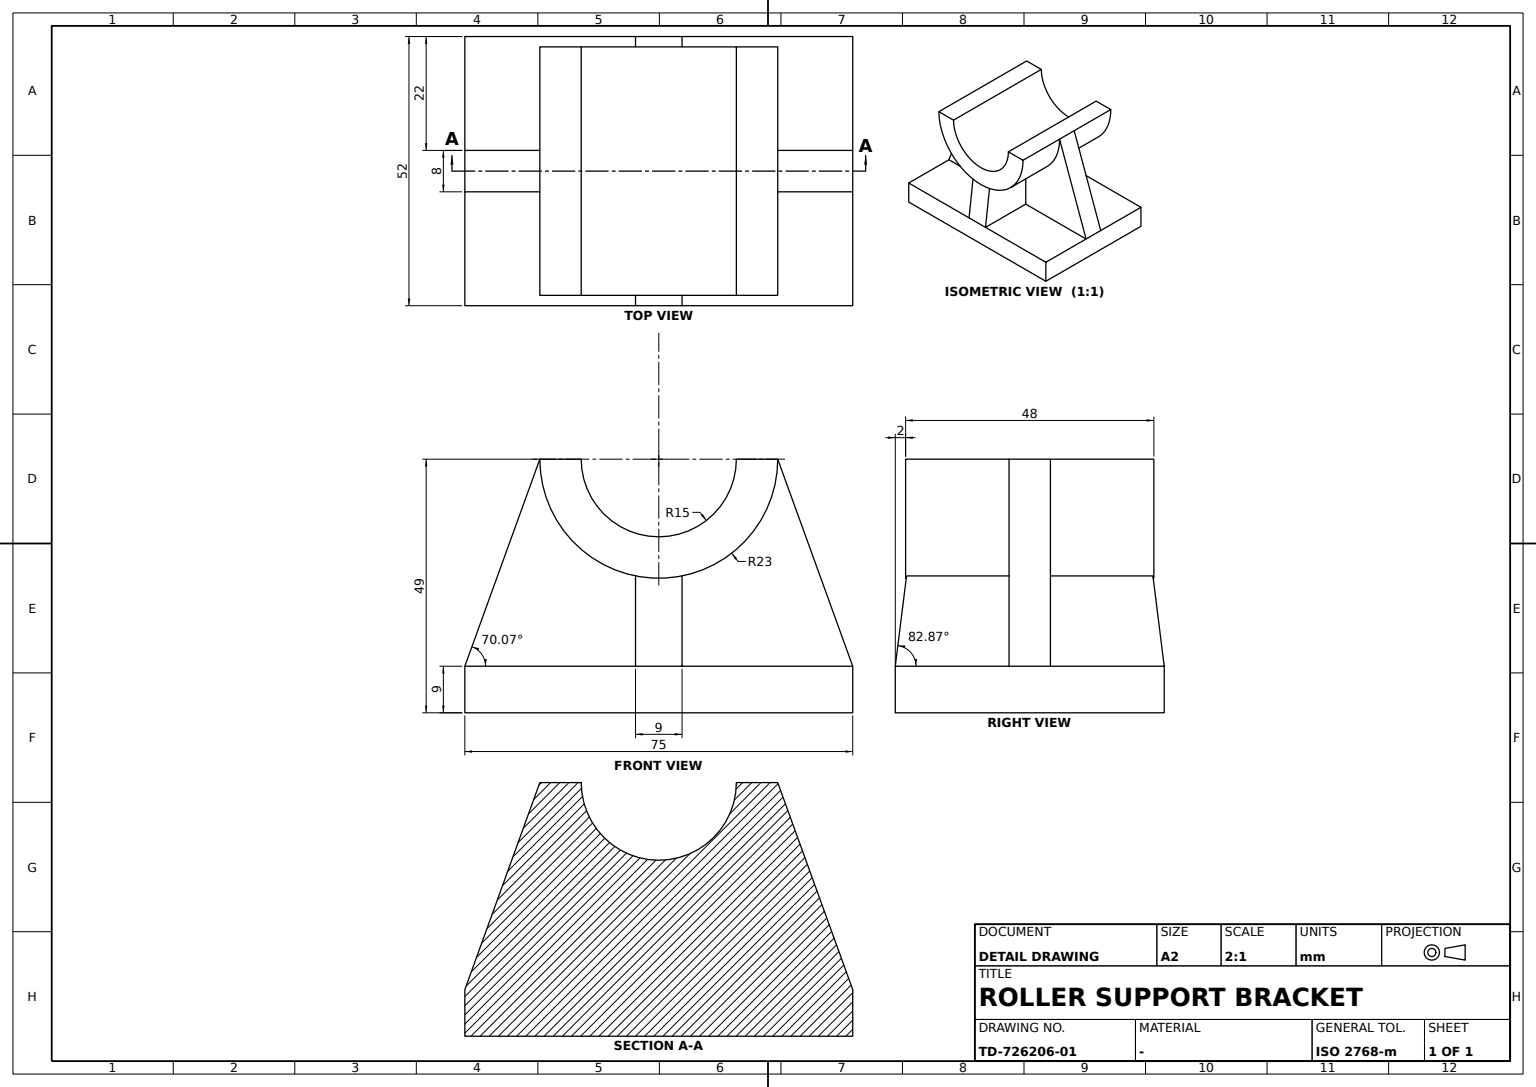
ISO-10303-21;
HEADER;
FILE_DESCRIPTION((''),'2;1');
FILE_NAME('','',(''),(''),'','','');
FILE_SCHEMA(('AUTOMOTIVE_DESIGN'));
ENDSEC;
DATA;
#1=APPLICATION_CONTEXT('');
#2=PRODUCT_CONTEXT('',#1,'mechanical');
#3=PRODUCT('','','',(#2));
#4=PRODUCT_DEFINITION_FORMATION('','',#3);
#5=PRODUCT_DEFINITION_CONTEXT('',#1,'design');
#6=PRODUCT_DEFINITION('','',#4,#5);
#7=PRODUCT_DEFINITION_SHAPE('','',#6);
#8=(LENGTH_UNIT()NAMED_UNIT(*)SI_UNIT(.MILLI.,.METRE.));
#9=(NAMED_UNIT(*)PLANE_ANGLE_UNIT()SI_UNIT($,.RADIAN.));
#10=(NAMED_UNIT(*)SI_UNIT($,.STERADIAN.)SOLID_ANGLE_UNIT());
#11=UNCERTAINTY_MEASURE_WITH_UNIT(LENGTH_MEASURE(0.005),#8,'distance_accuracy_value','');
#12=(GEOMETRIC_REPRESENTATION_CONTEXT(3)GLOBAL_UNCERTAINTY_ASSIGNED_CONTEXT((#11))GLOBAL_UNIT_ASSIGNED_CONTEXT((#8,#9,#10))REPRESENTATION_CONTEXT('',''));
#13=CARTESIAN_POINT('',(-4.,-37.5,4.5));
#14=VERTEX_POINT('',#13);
#15=CARTESIAN_POINT('',(4.,-37.5,4.5));
#16=VERTEX_POINT('',#15);
#17=CARTESIAN_POINT('',(0.,-37.5,4.5));
#18=DIRECTION('',(1.,0.,0.));
#19=VECTOR('',#18,1000.);
#20=LINE('',#17,#19);
#21=EDGE_CURVE('',#14,#16,#20,.T.);
#22=ORIENTED_EDGE('',*,*,#21,.T.);
#23=CARTESIAN_POINT('',(4.,-23.,44.5));
#24=VERTEX_POINT('',#23);
#25=CARTESIAN_POINT('',(4.,-34.586383,12.537564));
#26=DIRECTION('',(0.,-0.340799324,-0.940136065));
#27=VECTOR('',#26,1000.);
#28=LINE('',#25,#27);
#29=EDGE_CURVE('',#24,#16,#28,.T.);
#30=ORIENTED_EDGE('',*,*,#29,.F.);
#31=CARTESIAN_POINT('',(-4.,-23.,44.5));
#32=VERTEX_POINT('',#31);
#33=CARTESIAN_POINT('',(0.,-23.,44.5));
#34=LINE('',#33,#19);
#35=EDGE_CURVE('',#32,#24,#34,.T.);
#36=ORIENTED_EDGE('',*,*,#35,.F.);
#37=CARTESIAN_POINT('',(-4.,-34.586383,12.537564));
#38=LINE('',#37,#27);
#39=EDGE_CURVE('',#32,#14,#38,.T.);
#40=ORIENTED_EDGE('',*,*,#39,.T.);
#41=EDGE_LOOP('',(#22,#30,#36,#40));
#42=FACE_BOUND('',#41,.T.);
#43=DIRECTION('',(0.,-0.940136065,0.340799324));
#44=AXIS2_PLACEMENT_3D('',#33,#43,#26);
#45=PLANE('',#44);
#46=ADVANCED_FACE('',(#42),#45,.T.);
#47=CARTESIAN_POINT('',(24.,-15.,44.5));
#48=VERTEX_POINT('',#47);
#49=CARTESIAN_POINT('',(24.,15.,44.5));
#50=VERTEX_POINT('',#49);
#51=CARTESIAN_POINT('',(24.,0.,44.5));
#52=DIRECTION('',(0.,0.,-1.));
#53=AXIS2_PLACEMENT_3D('',#51,#18,#52);
#54=CIRCLE('',#53,15.);
#55=EDGE_CURVE('',#48,#50,#54,.T.);
#56=ORIENTED_EDGE('',*,*,#55,.T.);
#57=CARTESIAN_POINT('',(-24.,15.,44.5));
#58=VERTEX_POINT('',#57);
#59=LINE('',#57,#19);
#60=EDGE_CURVE('',#58,#50,#59,.T.);
#61=ORIENTED_EDGE('',*,*,#60,.F.);
#62=CARTESIAN_POINT('',(-24.,-15.,44.5));
#63=VERTEX_POINT('',#62);
#64=CARTESIAN_POINT('',(-24.,0.,44.5));
#65=AXIS2_PLACEMENT_3D('',#64,#18,#52);
#66=CIRCLE('',#65,15.);
#67=EDGE_CURVE('',#63,#58,#66,.T.);
#68=ORIENTED_EDGE('',*,*,#67,.F.);
#69=LINE('',#62,#19);
#70=EDGE_CURVE('',#63,#48,#69,.T.);
#71=ORIENTED_EDGE('',*,*,#70,.T.);
#72=EDGE_LOOP('',(#56,#61,#68,#71));
#73=FACE_BOUND('',#72,.T.);
#74=CARTESIAN_POINT('',(0.,0.,44.5));
#75=DIRECTION('',(0.,1.,0.));
#76=AXIS2_PLACEMENT_3D('',#74,#18,#75);
#77=CYLINDRICAL_SURFACE('',#76,15.);
#78=ADVANCED_FACE('',(#73),#77,.F.);
#79=CARTESIAN_POINT('',(4.,4.5,21.944513));
#80=VERTEX_POINT('',#79);
#81=CARTESIAN_POINT('',(4.,4.5,4.5));
#82=VERTEX_POINT('',#81);
#83=CARTESIAN_POINT('',(4.,4.5,0.));
#84=VECTOR('',#52,1000.);
#85=LINE('',#83,#84);
#86=EDGE_CURVE('',#80,#82,#85,.T.);
#87=ORIENTED_EDGE('',*,*,#86,.F.);
#88=CARTESIAN_POINT('',(23.819436,4.5,21.944513));
#89=VERTEX_POINT('',#88);
#90=LINE('',#79,#19);
#91=EDGE_CURVE('',#80,#89,#90,.T.);
#92=ORIENTED_EDGE('',*,*,#91,.T.);
#93=CARTESIAN_POINT('',(26.,4.5,4.5));
#94=VERTEX_POINT('',#93);
#95=CARTESIAN_POINT('',(24.,4.5,20.5));
#96=DIRECTION('',(0.124034735,0.,-0.992277877));
#97=VECTOR('',#96,1000.);
#98=LINE('',#95,#97);
#99=EDGE_CURVE('',#89,#94,#98,.T.);
#100=ORIENTED_EDGE('',*,*,#99,.T.);
#101=CARTESIAN_POINT('',(0.,4.5,4.5));
#102=LINE('',#101,#19);
#103=EDGE_CURVE('',#82,#94,#102,.T.);
#104=ORIENTED_EDGE('',*,*,#103,.F.);
#105=EDGE_LOOP('',(#87,#92,#100,#104));
#106=FACE_BOUND('',#105,.T.);
#107=CARTESIAN_POINT('',(0.,4.5,0.));
#108=DIRECTION('',(-1.,0.,0.));
#109=AXIS2_PLACEMENT_3D('',#107,#75,#108);
#110=PLANE('',#109);
#111=ADVANCED_FACE('',(#106),#110,.T.);
#112=CARTESIAN_POINT('',(26.,37.5,4.5));
#113=VERTEX_POINT('',#112);
#114=CARTESIAN_POINT('',(4.,37.5,4.5));
#115=VERTEX_POINT('',#114);
#116=CARTESIAN_POINT('',(0.,37.5,4.5));
#117=VECTOR('',#108,1000.);
#118=LINE('',#116,#117);
#119=EDGE_CURVE('',#113,#115,#118,.T.);
#120=ORIENTED_EDGE('',*,*,#119,.T.);
#121=CARTESIAN_POINT('',(4.,0.,4.5));
#122=DIRECTION('',(0.,-1.,0.));
#123=VECTOR('',#122,1000.);
#124=LINE('',#121,#123);
#125=EDGE_CURVE('',#115,#82,#124,.T.);
#126=ORIENTED_EDGE('',*,*,#125,.T.);
#127=ORIENTED_EDGE('',*,*,#103,.T.);
#128=CARTESIAN_POINT('',(26.,-37.5,4.5));
#129=VECTOR('',#75,1000.);
#130=LINE('',#128,#129);
#131=EDGE_CURVE('',#94,#113,#130,.T.);
#132=ORIENTED_EDGE('',*,*,#131,.T.);
#133=EDGE_LOOP('',(#120,#126,#127,#132));
#134=FACE_BOUND('',#133,.T.);
#135=DIRECTION('',(0.,0.,1.));
#136=AXIS2_PLACEMENT_3D('',#17,#135,#75);
#137=PLANE('',#136);
#138=ADVANCED_FACE('',(#134),#137,.T.);
#139=CARTESIAN_POINT('',(-24.,23.,44.5));
#140=VERTEX_POINT('',#139);
#141=CARTESIAN_POINT('',(-4.,23.,44.5));
#142=VERTEX_POINT('',#141);
#143=LINE('',#139,#19);
#144=EDGE_CURVE('',#140,#142,#143,.T.);
#145=ORIENTED_EDGE('',*,*,#144,.T.);
#146=CARTESIAN_POINT('',(-4.,4.5,21.944513));
#147=VERTEX_POINT('',#146);
#148=CARTESIAN_POINT('',(-4.,0.,44.5));
#149=AXIS2_PLACEMENT_3D('',#148,#18,#52);
#150=CIRCLE('',#149,23.);
#151=EDGE_CURVE('',#147,#142,#150,.T.);
#152=ORIENTED_EDGE('',*,*,#151,.F.);
#153=CARTESIAN_POINT('',(-23.819436,4.5,21.944513));
#154=VERTEX_POINT('',#153);
#155=LINE('',#153,#19);
#156=EDGE_CURVE('',#154,#147,#155,.T.);
#157=ORIENTED_EDGE('',*,*,#156,.F.);
#158=CARTESIAN_POINT('',(-23.819436,-4.5,21.944513));
#159=VERTEX_POINT('',#158);
#160=CARTESIAN_POINT('',(-21.,0.,44.5));
#161=DIRECTION('',(0.992277877,0.,-0.124034735));
#162=DIRECTION('',(0.124034735,0.,0.992277877));
#163=AXIS2_PLACEMENT_3D('',#160,#161,#162);
#164=ELLIPSE('',#163,23.178991,23.);
#165=EDGE_CURVE('',#154,#159,#164,.F.);
#166=ORIENTED_EDGE('',*,*,#165,.T.);
#167=CARTESIAN_POINT('',(-4.,-4.5,21.944513));
#168=VERTEX_POINT('',#167);
#169=LINE('',#158,#19);
#170=EDGE_CURVE('',#159,#168,#169,.T.);
#171=ORIENTED_EDGE('',*,*,#170,.T.);
#172=EDGE_CURVE('',#32,#168,#150,.T.);
#173=ORIENTED_EDGE('',*,*,#172,.F.);
#174=CARTESIAN_POINT('',(-24.,-23.,44.5));
#175=VERTEX_POINT('',#174);
#176=LINE('',#174,#19);
#177=EDGE_CURVE('',#175,#32,#176,.T.);
#178=ORIENTED_EDGE('',*,*,#177,.F.);
#179=CIRCLE('',#65,23.);
#180=EDGE_CURVE('',#175,#140,#179,.T.);
#181=ORIENTED_EDGE('',*,*,#180,.T.);
#182=EDGE_LOOP('',(#145,#152,#157,#166,#171,#173,#178,#181));
#183=FACE_BOUND('',#182,.T.);
#184=CYLINDRICAL_SURFACE('',#76,23.);
#185=ADVANCED_FACE('',(#183),#184,.T.);
#186=VERTEX_POINT('',#128);
#187=LINE('',#17,#117);
#188=EDGE_CURVE('',#186,#16,#187,.T.);
#189=ORIENTED_EDGE('',*,*,#188,.F.);
#190=CARTESIAN_POINT('',(26.,-4.5,4.5));
#191=VERTEX_POINT('',#190);
#192=EDGE_CURVE('',#186,#191,#130,.T.);
#193=ORIENTED_EDGE('',*,*,#192,.T.);
#194=CARTESIAN_POINT('',(4.,-4.5,4.5));
#195=VERTEX_POINT('',#194);
#196=CARTESIAN_POINT('',(0.,-4.5,4.5));
#197=LINE('',#196,#19);
#198=EDGE_CURVE('',#195,#191,#197,.T.);
#199=ORIENTED_EDGE('',*,*,#198,.F.);
#200=EDGE_CURVE('',#195,#16,#124,.T.);
#201=ORIENTED_EDGE('',*,*,#200,.T.);
#202=EDGE_LOOP('',(#189,#193,#199,#201));
#203=FACE_BOUND('',#202,.T.);
#204=ADVANCED_FACE('',(#203),#137,.T.);
#205=CARTESIAN_POINT('',(-26.,-4.5,4.5));
#206=VERTEX_POINT('',#205);
#207=CARTESIAN_POINT('',(-26.,4.5,4.5));
#208=VERTEX_POINT('',#207);
#209=CARTESIAN_POINT('',(-26.,0.,4.5));
#210=LINE('',#209,#129);
#211=EDGE_CURVE('',#206,#208,#210,.T.);
#212=ORIENTED_EDGE('',*,*,#211,.T.);
#213=CARTESIAN_POINT('',(-26.,37.5,4.5));
#214=VERTEX_POINT('',#213);
#215=CARTESIAN_POINT('',(-26.,-37.5,4.5));
#216=LINE('',#215,#129);
#217=EDGE_CURVE('',#208,#214,#216,.T.);
#218=ORIENTED_EDGE('',*,*,#217,.T.);
#219=CARTESIAN_POINT('',(-26.,37.5,-4.5));
#220=VERTEX_POINT('',#219);
#221=LINE('',#213,#84);
#222=EDGE_CURVE('',#214,#220,#221,.T.);
#223=ORIENTED_EDGE('',*,*,#222,.T.);
#224=CARTESIAN_POINT('',(-26.,-37.5,-4.5));
#225=VERTEX_POINT('',#224);
#226=LINE('',#219,#123);
#227=EDGE_CURVE('',#220,#225,#226,.T.);
#228=ORIENTED_EDGE('',*,*,#227,.T.);
#229=VERTEX_POINT('',#215);
#230=VECTOR('',#135,1000.);
#231=LINE('',#224,#230);
#232=EDGE_CURVE('',#225,#229,#231,.T.);
#233=ORIENTED_EDGE('',*,*,#232,.T.);
#234=EDGE_CURVE('',#229,#206,#216,.T.);
#235=ORIENTED_EDGE('',*,*,#234,.T.);
#236=EDGE_LOOP('',(#212,#218,#223,#228,#233,#235));
#237=FACE_BOUND('',#236,.T.);
#238=CARTESIAN_POINT('',(-26.,0.,0.));
#239=AXIS2_PLACEMENT_3D('',#238,#18,#75);
#240=PLANE('',#239);
#241=ADVANCED_FACE('',(#237),#240,.F.);
#242=ORIENTED_EDGE('',*,*,#217,.F.);
#243=CARTESIAN_POINT('',(-4.,4.5,4.5));
#244=VERTEX_POINT('',#243);
#245=EDGE_CURVE('',#208,#244,#102,.T.);
#246=ORIENTED_EDGE('',*,*,#245,.T.);
#247=CARTESIAN_POINT('',(-4.,37.5,4.5));
#248=VERTEX_POINT('',#247);
#249=CARTESIAN_POINT('',(-4.,0.,4.5));
#250=LINE('',#249,#123);
#251=EDGE_CURVE('',#248,#244,#250,.T.);
#252=ORIENTED_EDGE('',*,*,#251,.F.);
#253=EDGE_CURVE('',#248,#214,#118,.T.);
#254=ORIENTED_EDGE('',*,*,#253,.T.);
#255=EDGE_LOOP('',(#242,#246,#252,#254));
#256=FACE_BOUND('',#255,.T.);
#257=ADVANCED_FACE('',(#256),#137,.T.);
#258=CARTESIAN_POINT('',(4.,-4.5,21.944513));
#259=VERTEX_POINT('',#258);
#260=CARTESIAN_POINT('',(4.,-4.5,0.));
#261=LINE('',#260,#84);
#262=EDGE_CURVE('',#259,#195,#261,.T.);
#263=ORIENTED_EDGE('',*,*,#262,.T.);
#264=ORIENTED_EDGE('',*,*,#198,.T.);
#265=CARTESIAN_POINT('',(23.819436,-4.5,21.944513));
#266=VERTEX_POINT('',#265);
#267=CARTESIAN_POINT('',(24.,-4.5,20.5));
#268=LINE('',#267,#97);
#269=EDGE_CURVE('',#266,#191,#268,.T.);
#270=ORIENTED_EDGE('',*,*,#269,.F.);
#271=LINE('',#258,#19);
#272=EDGE_CURVE('',#259,#266,#271,.T.);
#273=ORIENTED_EDGE('',*,*,#272,.F.);
#274=EDGE_LOOP('',(#263,#264,#270,#273));
#275=FACE_BOUND('',#274,.T.);
#276=CARTESIAN_POINT('',(0.,-4.5,0.));
#277=AXIS2_PLACEMENT_3D('',#276,#75,#108);
#278=PLANE('',#277);
#279=ADVANCED_FACE('',(#275),#278,.F.);
#280=CARTESIAN_POINT('',(-4.,-4.5,4.5));
#281=VERTEX_POINT('',#280);
#282=EDGE_CURVE('',#206,#281,#197,.T.);
#283=ORIENTED_EDGE('',*,*,#282,.T.);
#284=CARTESIAN_POINT('',(-4.,-4.5,0.));
#285=LINE('',#284,#84);
#286=EDGE_CURVE('',#168,#281,#285,.T.);
#287=ORIENTED_EDGE('',*,*,#286,.F.);
#288=ORIENTED_EDGE('',*,*,#170,.F.);
#289=CARTESIAN_POINT('',(-24.,-4.5,20.5));
#290=VECTOR('',#162,1000.);
#291=LINE('',#289,#290);
#292=EDGE_CURVE('',#206,#159,#291,.T.);
#293=ORIENTED_EDGE('',*,*,#292,.F.);
#294=EDGE_LOOP('',(#283,#287,#288,#293));
#295=FACE_BOUND('',#294,.T.);
#296=ADVANCED_FACE('',(#295),#278,.F.);
#297=ORIENTED_EDGE('',*,*,#165,.F.);
#298=CARTESIAN_POINT('',(-26.153846,4.5,3.269231));
#299=DIRECTION('',(-0.124034735,0.,-0.992277877));
#300=VECTOR('',#299,1000.);
#301=LINE('',#298,#300);
#302=EDGE_CURVE('',#154,#208,#301,.T.);
#303=ORIENTED_EDGE('',*,*,#302,.T.);
#304=ORIENTED_EDGE('',*,*,#211,.F.);
#305=ORIENTED_EDGE('',*,*,#292,.T.);
#306=EDGE_LOOP('',(#297,#303,#304,#305));
#307=FACE_BOUND('',#306,.T.);
#308=CARTESIAN_POINT('',(-24.,0.,20.5));
#309=AXIS2_PLACEMENT_3D('',#308,#161,#162);
#310=PLANE('',#309);
#311=ADVANCED_FACE('',(#307),#310,.F.);
#312=CARTESIAN_POINT('',(4.,23.,44.5));
#313=VERTEX_POINT('',#312);
#314=CARTESIAN_POINT('',(4.,34.586383,12.537564));
#315=DIRECTION('',(0.,0.340799324,-0.940136065));
#316=VECTOR('',#315,1000.);
#317=LINE('',#314,#316);
#318=EDGE_CURVE('',#313,#115,#317,.T.);
#319=ORIENTED_EDGE('',*,*,#318,.T.);
#320=LINE('',#116,#19);
#321=EDGE_CURVE('',#248,#115,#320,.T.);
#322=ORIENTED_EDGE('',*,*,#321,.F.);
#323=CARTESIAN_POINT('',(-4.,34.586383,12.537564));
#324=LINE('',#323,#316);
#325=EDGE_CURVE('',#142,#248,#324,.T.);
#326=ORIENTED_EDGE('',*,*,#325,.F.);
#327=CARTESIAN_POINT('',(0.,23.,44.5));
#328=LINE('',#327,#19);
#329=EDGE_CURVE('',#142,#313,#328,.T.);
#330=ORIENTED_EDGE('',*,*,#329,.T.);
#331=EDGE_LOOP('',(#319,#322,#326,#330));
#332=FACE_BOUND('',#331,.T.);
#333=DIRECTION('',(0.,-0.940136065,-0.340799324));
#334=AXIS2_PLACEMENT_3D('',#327,#333,#315);
#335=PLANE('',#334);
#336=ADVANCED_FACE('',(#332),#335,.F.);
#337=ORIENTED_EDGE('',*,*,#29,.T.);
#338=ORIENTED_EDGE('',*,*,#200,.F.);
#339=ORIENTED_EDGE('',*,*,#262,.F.);
#340=CARTESIAN_POINT('',(4.,0.,44.5));
#341=AXIS2_PLACEMENT_3D('',#340,#18,#52);
#342=CIRCLE('',#341,23.);
#343=EDGE_CURVE('',#24,#259,#342,.T.);
#344=ORIENTED_EDGE('',*,*,#343,.F.);
#345=EDGE_LOOP('',(#337,#338,#339,#344));
#346=FACE_BOUND('',#345,.T.);
#347=CARTESIAN_POINT('',(4.,0.,0.));
#348=AXIS2_PLACEMENT_3D('',#347,#18,#75);
#349=PLANE('',#348);
#350=ADVANCED_FACE('',(#346),#349,.T.);
#351=CARTESIAN_POINT('',(26.,0.,4.5));
#352=LINE('',#351,#123);
#353=EDGE_CURVE('',#94,#191,#352,.T.);
#354=ORIENTED_EDGE('',*,*,#353,.T.);
#355=ORIENTED_EDGE('',*,*,#192,.F.);
#356=CARTESIAN_POINT('',(26.,-37.5,-4.5));
#357=VERTEX_POINT('',#356);
#358=LINE('',#356,#230);
#359=EDGE_CURVE('',#357,#186,#358,.T.);
#360=ORIENTED_EDGE('',*,*,#359,.F.);
#361=CARTESIAN_POINT('',(26.,37.5,-4.5));
#362=VERTEX_POINT('',#361);
#363=LINE('',#361,#123);
#364=EDGE_CURVE('',#362,#357,#363,.T.);
#365=ORIENTED_EDGE('',*,*,#364,.F.);
#366=LINE('',#112,#84);
#367=EDGE_CURVE('',#113,#362,#366,.T.);
#368=ORIENTED_EDGE('',*,*,#367,.F.);
#369=ORIENTED_EDGE('',*,*,#131,.F.);
#370=EDGE_LOOP('',(#354,#355,#360,#365,#368,#369));
#371=FACE_BOUND('',#370,.T.);
#372=CARTESIAN_POINT('',(26.,0.,0.));
#373=AXIS2_PLACEMENT_3D('',#372,#18,#75);
#374=PLANE('',#373);
#375=ADVANCED_FACE('',(#371),#374,.T.);
#376=ORIENTED_EDGE('',*,*,#125,.F.);
#377=ORIENTED_EDGE('',*,*,#318,.F.);
#378=EDGE_CURVE('',#80,#313,#342,.T.);
#379=ORIENTED_EDGE('',*,*,#378,.F.);
#380=ORIENTED_EDGE('',*,*,#86,.T.);
#381=EDGE_LOOP('',(#376,#377,#379,#380));
#382=FACE_BOUND('',#381,.T.);
#383=ADVANCED_FACE('',(#382),#349,.T.);
#384=ORIENTED_EDGE('',*,*,#234,.F.);
#385=EDGE_CURVE('',#14,#229,#187,.T.);
#386=ORIENTED_EDGE('',*,*,#385,.F.);
#387=EDGE_CURVE('',#281,#14,#250,.T.);
#388=ORIENTED_EDGE('',*,*,#387,.F.);
#389=ORIENTED_EDGE('',*,*,#282,.F.);
#390=EDGE_LOOP('',(#384,#386,#388,#389));
#391=FACE_BOUND('',#390,.T.);
#392=ADVANCED_FACE('',(#391),#137,.T.);
#393=CARTESIAN_POINT('',(24.,-23.,44.5));
#394=VERTEX_POINT('',#393);
#395=LINE('',#51,#129);
#396=EDGE_CURVE('',#394,#48,#395,.T.);
#397=ORIENTED_EDGE('',*,*,#396,.T.);
#398=ORIENTED_EDGE('',*,*,#70,.F.);
#399=LINE('',#64,#129);
#400=EDGE_CURVE('',#175,#63,#399,.T.);
#401=ORIENTED_EDGE('',*,*,#400,.F.);
#402=ORIENTED_EDGE('',*,*,#177,.T.);
#403=ORIENTED_EDGE('',*,*,#35,.T.);
#404=LINE('',#23,#19);
#405=EDGE_CURVE('',#24,#394,#404,.T.);
#406=ORIENTED_EDGE('',*,*,#405,.T.);
#407=EDGE_LOOP('',(#397,#398,#401,#402,#403,#406));
#408=FACE_BOUND('',#407,.T.);
#409=AXIS2_PLACEMENT_3D('',#33,#52,#75);
#410=PLANE('',#409);
#411=ADVANCED_FACE('',(#408),#410,.F.);
#412=ORIENTED_EDGE('',*,*,#180,.F.);
#413=ORIENTED_EDGE('',*,*,#400,.T.);
#414=ORIENTED_EDGE('',*,*,#67,.T.);
#415=EDGE_CURVE('',#58,#140,#399,.T.);
#416=ORIENTED_EDGE('',*,*,#415,.T.);
#417=EDGE_LOOP('',(#412,#413,#414,#416));
#418=FACE_BOUND('',#417,.T.);
#419=CARTESIAN_POINT('',(-24.,0.,0.));
#420=AXIS2_PLACEMENT_3D('',#419,#18,#75);
#421=PLANE('',#420);
#422=ADVANCED_FACE('',(#418),#421,.F.);
#423=CARTESIAN_POINT('',(24.,23.,44.5));
#424=VERTEX_POINT('',#423);
#425=CIRCLE('',#53,23.);
#426=EDGE_CURVE('',#394,#424,#425,.T.);
#427=ORIENTED_EDGE('',*,*,#426,.T.);
#428=EDGE_CURVE('',#50,#424,#395,.T.);
#429=ORIENTED_EDGE('',*,*,#428,.F.);
#430=ORIENTED_EDGE('',*,*,#55,.F.);
#431=ORIENTED_EDGE('',*,*,#396,.F.);
#432=EDGE_LOOP('',(#427,#429,#430,#431));
#433=FACE_BOUND('',#432,.T.);
#434=CARTESIAN_POINT('',(24.,0.,0.));
#435=AXIS2_PLACEMENT_3D('',#434,#18,#75);
#436=PLANE('',#435);
#437=ADVANCED_FACE('',(#433),#436,.T.);
#438=ORIENTED_EDGE('',*,*,#387,.T.);
#439=ORIENTED_EDGE('',*,*,#39,.F.);
#440=ORIENTED_EDGE('',*,*,#172,.T.);
#441=ORIENTED_EDGE('',*,*,#286,.T.);
#442=EDGE_LOOP('',(#438,#439,#440,#441));
#443=FACE_BOUND('',#442,.T.);
#444=CARTESIAN_POINT('',(-4.,0.,0.));
#445=AXIS2_PLACEMENT_3D('',#444,#18,#75);
#446=PLANE('',#445);
#447=ADVANCED_FACE('',(#443),#446,.F.);
#448=ORIENTED_EDGE('',*,*,#245,.F.);
#449=ORIENTED_EDGE('',*,*,#302,.F.);
#450=ORIENTED_EDGE('',*,*,#156,.T.);
#451=CARTESIAN_POINT('',(-4.,4.5,0.));
#452=LINE('',#451,#84);
#453=EDGE_CURVE('',#147,#244,#452,.T.);
#454=ORIENTED_EDGE('',*,*,#453,.T.);
#455=EDGE_LOOP('',(#448,#449,#450,#454));
#456=FACE_BOUND('',#455,.T.);
#457=ADVANCED_FACE('',(#456),#110,.T.);
#458=CARTESIAN_POINT('',(0.,37.5,-4.5));
#459=LINE('',#458,#117);
#460=EDGE_CURVE('',#362,#220,#459,.T.);
#461=ORIENTED_EDGE('',*,*,#460,.F.);
#462=ORIENTED_EDGE('',*,*,#364,.T.);
#463=CARTESIAN_POINT('',(0.,-37.5,-4.5));
#464=LINE('',#463,#117);
#465=EDGE_CURVE('',#357,#225,#464,.T.);
#466=ORIENTED_EDGE('',*,*,#465,.T.);
#467=ORIENTED_EDGE('',*,*,#227,.F.);
#468=EDGE_LOOP('',(#461,#462,#466,#467));
#469=FACE_BOUND('',#468,.T.);
#470=AXIS2_PLACEMENT_3D('',#458,#52,#122);
#471=PLANE('',#470);
#472=ADVANCED_FACE('',(#469),#471,.T.);
#473=ORIENTED_EDGE('',*,*,#465,.F.);
#474=ORIENTED_EDGE('',*,*,#359,.T.);
#475=ORIENTED_EDGE('',*,*,#188,.T.);
#476=ORIENTED_EDGE('',*,*,#21,.F.);
#477=ORIENTED_EDGE('',*,*,#385,.T.);
#478=ORIENTED_EDGE('',*,*,#232,.F.);
#479=EDGE_LOOP('',(#473,#474,#475,#476,#477,#478));
#480=FACE_BOUND('',#479,.T.);
#481=AXIS2_PLACEMENT_3D('',#463,#122,#135);
#482=PLANE('',#481);
#483=ADVANCED_FACE('',(#480),#482,.T.);
#484=ORIENTED_EDGE('',*,*,#405,.F.);
#485=ORIENTED_EDGE('',*,*,#343,.T.);
#486=ORIENTED_EDGE('',*,*,#272,.T.);
#487=CARTESIAN_POINT('',(21.,0.,44.5));
#488=DIRECTION('',(-0.992277877,0.,-0.124034735));
#489=AXIS2_PLACEMENT_3D('',#487,#488,#96);
#490=ELLIPSE('',#489,23.178991,23.);
#491=EDGE_CURVE('',#266,#89,#490,.F.);
#492=ORIENTED_EDGE('',*,*,#491,.T.);
#493=ORIENTED_EDGE('',*,*,#91,.F.);
#494=ORIENTED_EDGE('',*,*,#378,.T.);
#495=LINE('',#312,#19);
#496=EDGE_CURVE('',#313,#424,#495,.T.);
#497=ORIENTED_EDGE('',*,*,#496,.T.);
#498=ORIENTED_EDGE('',*,*,#426,.F.);
#499=EDGE_LOOP('',(#484,#485,#486,#492,#493,#494,#497,#498));
#500=FACE_BOUND('',#499,.T.);
#501=ADVANCED_FACE('',(#500),#184,.T.);
#502=ORIENTED_EDGE('',*,*,#253,.F.);
#503=ORIENTED_EDGE('',*,*,#321,.T.);
#504=ORIENTED_EDGE('',*,*,#119,.F.);
#505=ORIENTED_EDGE('',*,*,#367,.T.);
#506=ORIENTED_EDGE('',*,*,#460,.T.);
#507=ORIENTED_EDGE('',*,*,#222,.F.);
#508=EDGE_LOOP('',(#502,#503,#504,#505,#506,#507));
#509=FACE_BOUND('',#508,.T.);
#510=AXIS2_PLACEMENT_3D('',#116,#75,#52);
#511=PLANE('',#510);
#512=ADVANCED_FACE('',(#509),#511,.T.);
#513=ORIENTED_EDGE('',*,*,#496,.F.);
#514=ORIENTED_EDGE('',*,*,#329,.F.);
#515=ORIENTED_EDGE('',*,*,#144,.F.);
#516=ORIENTED_EDGE('',*,*,#415,.F.);
#517=ORIENTED_EDGE('',*,*,#60,.T.);
#518=ORIENTED_EDGE('',*,*,#428,.T.);
#519=EDGE_LOOP('',(#513,#514,#515,#516,#517,#518));
#520=FACE_BOUND('',#519,.T.);
#521=ADVANCED_FACE('',(#520),#410,.F.);
#522=ORIENTED_EDGE('',*,*,#325,.T.);
#523=ORIENTED_EDGE('',*,*,#251,.T.);
#524=ORIENTED_EDGE('',*,*,#453,.F.);
#525=ORIENTED_EDGE('',*,*,#151,.T.);
#526=EDGE_LOOP('',(#522,#523,#524,#525));
#527=FACE_BOUND('',#526,.T.);
#528=ADVANCED_FACE('',(#527),#446,.F.);
#529=ORIENTED_EDGE('',*,*,#269,.T.);
#530=ORIENTED_EDGE('',*,*,#353,.F.);
#531=ORIENTED_EDGE('',*,*,#99,.F.);
#532=ORIENTED_EDGE('',*,*,#491,.F.);
#533=EDGE_LOOP('',(#529,#530,#531,#532));
#534=FACE_BOUND('',#533,.T.);
#535=CARTESIAN_POINT('',(24.,0.,20.5));
#536=DIRECTION('',(-0.124034735,0.,0.992277877));
#537=AXIS2_PLACEMENT_3D('',#535,#488,#536);
#538=PLANE('',#537);
#539=ADVANCED_FACE('',(#534),#538,.F.);
#540=CLOSED_SHELL('',(#46,#78,#111,#138,#185,#204,#241,#257,#279,#296,#311,#336,#350,#375,#383,#392,#411,#422,#437,#447,#457,#472,#483,#501,#512,#521,#528,#539));
#541=MANIFOLD_SOLID_BREP('',#540);
#542=ADVANCED_BREP_SHAPE_REPRESENTATION('',(#541),#12);
#543=SHAPE_DEFINITION_REPRESENTATION(#7,#542);
ENDSEC;
END-ISO-10303-21;
